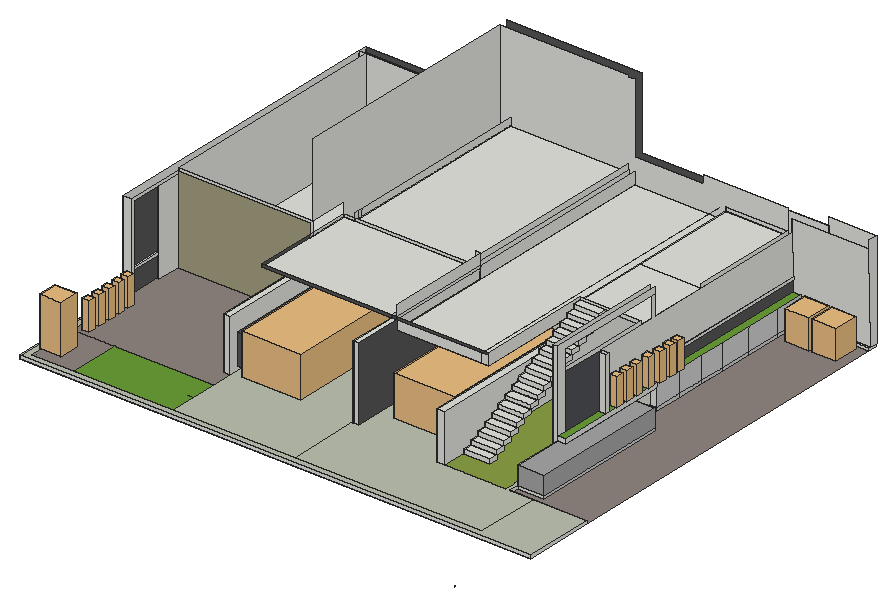
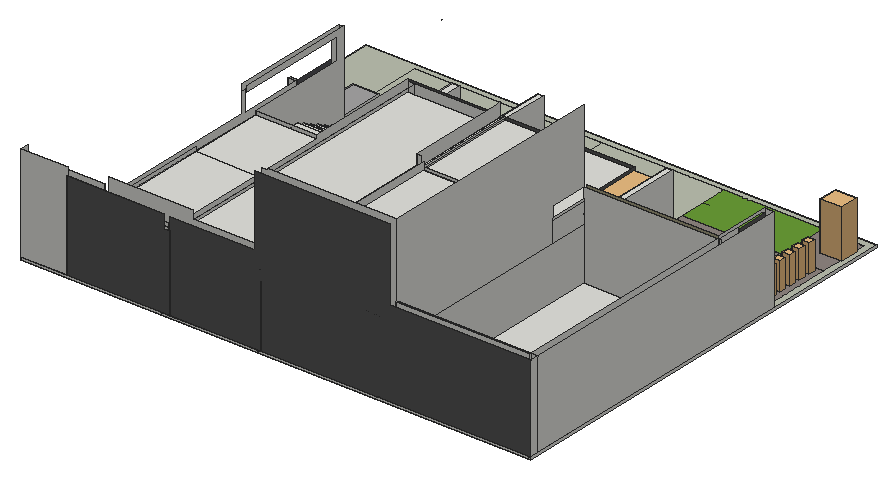
# SketchUp Ruby script. Lengths in inches.
U = 1.inch
M = Sketchup.active_model
def pt(a) = Geom::Point3d.new(a.map { |v| v * U })
def face(e, loops, mat)
  f = e.add_face(loops[0].map { |a| pt(a) })
  loops[1..].each { |l| e.add_face(l.map { |a| pt(a) }).erase! }
  f.material = f.back_material = mat if mat
  f
end
# faces: each face lists its corners as indices into pts; further lists are holes
def faces(e, pts, list, mat = nil) = list.each { |f| face(e, (f[0].is_a?(Array) ? f : [f]).map { |l| l.map { |i| pts[i] } }, mat) }
# xy, xz, yz: faces in a plane at the given z, y or x. An outline is a flat list of corners, or four numbers for a rectangle; further outlines are holes
def ring(l) = l.size == 4 ? [[l[0], l[1]], [l[2], l[1]], [l[2], l[3]], [l[0], l[3]]] : l.each_slice(2).to_a
def flat(e, list, mat, &to3) = list.each { |f| face(e, (f[0].is_a?(Array) ? f : [f]).map { |l| ring(l).map { |u, v| to3.(u, v) } }, mat) }
def xy(e, z, list, mat = nil) = flat(e, list, mat) { |x, y| [x, y, z] }
def xz(e, y, list, mat = nil) = flat(e, list, mat) { |x, z| [x, y, z] }
def yz(e, x, list, mat = nil) = flat(e, list, mat) { |y, z| [x, y, z] }
def lines(e, pts, list) = list.each { |a, b| e.add_line(pt(pts[a]), pt(pts[b])) }
# prism: a flat outline (further loops are holes) pulled along v
def prism(e, loops, v, mat = nil)
  f = face(e, loops, mat); d = Geom::Vector3d.new(v.map { |x| x * U })
  f.pushpull(f.normal.samedirection?(d) ? d.length : -d.length)
end
def box(e, o, s, mat = nil) = prism(e, [[o, [o[0] + s[0], o[1], o[2]], [o[0] + s[0], o[1] + s[1], o[2]], [o[0], o[1] + s[1], o[2]]]], [0, 0, s[2]], mat)
def at(x, y, z, deg = 0) = Geom::Transformation.translation(pt([x, y, z])) * Geom::Transformation.rotation(ORIGIN, Z_AXIS, deg.degrees)
def axes(o, x, y, z) = Geom::Transformation.new([*x, 0, *y, 0, *z, 0, *pt(o).to_a, 1])
def part(name) = M.definitions.add(name)
# library, detail: a bought-in or finely detailed component or shape, given as its bounding box
def library(name, o, s) = part(name).tap { |d| box(d.entities, o, s) }
def detail(e, o, s) = box(e.add_group.entities, o, s)
def put(e, d, t, mat = nil) = e.add_instance(d, t).tap { |i| i.material = mat if mat }
def group(e, t, mat = nil) = e.add_group.tap { |g| g.transformation = t; g.material = mat if mat }.entities
root = M.entities
M.materials.add("[Blinds Roman Hobbled Blue]").color = [81, 82, 87]
M.materials.add("[Carrera Marble]").color = [207, 207, 207]
M.materials.add("[Color M06]").color = [86, 86, 86]
M.materials.add("[Grass Dark Green]").color = [106, 157, 55]
M.materials.add("[Grass Light Green]").color = [138, 158, 69]
M.materials.add("[Groundcover Rock Crushed Multi]").color = [143, 133, 129]
M.materials.add("[Pavers with Grass Brick]").color = [187, 192, 176]
M.materials.add("[Stone Coursed Rough]").color = [165, 160, 130]
M.materials.add("[Stone Vein Gray]").color = [166, 165, 165]
c1 = library("PLANTS 75\#1",[-17.06,-18.11,0],[33.69,34.67,40.66])
c2 = library("bmw m6",[0,0,0],[74.56,175.18,49.66])
c3 = library("MERCEDES LIGHT",[-74.97,-97.73,0.18],[82.22,195.9,56.22])
c4 = library("araç",[-7.9,-14.14,0],[84.07,190.26,56.29])
c5 = part("Group\#4")
box(c5.entities,[0,0,0],[36,12,6])
c6 = library("PLANTS 75",[-17.8,-11.72,0],[29.52,26.34,67.21])
c7 = library("Plant Pot 02 - Garden Croton",[-1.84,-1.8,0],[9.84,9.84,38.82])
xy(root,0,[[710.71,0,710.77,0,710.83,0.04,710.85,0.0625,710.86,0.09,710.86,0.16,710.85,0.1875,710.83,0.21,710.77,0.25,710.71,0.25,710.65,0.21,710.63,0.1875,710.62,0.16,710.61,0.125,710.62,0.09,710.63,0.0625,710.65,0.04],[27.5625,99.87,27.5625,699.87,736.75,699.87,736.75,688.37,640,688.37,640,687.87,39.5625,687.87,39.5625,111.87,736.75,111.87,736.75,99.87],[39.5625,111.87,39.5625,687.87,640,687.87,640,440.86,629.0625,440.86,629.0625,403.96,665.5,403.96,665.5,211.52,629.0625,211.52,629.0625,198.37,736.75,198.37,736.75,111.87],[640,687.87,736.75,688.37]])
xy(root,0,[[629.0625,198.37,736.75,198.37,736.75,687.87,640,687.87,640,440.86,629.0625,440.86,629.0625,403.96,665.5,403.96,665.5,211.52,629.0625,211.52]],"[Groundcover Rock Crushed Multi]")
xy(root,3.4375,[[404.1875,699.87,415.125,700.56]])
xy(root,4,[[223,208.68,232,208.68,232,418.01,238,418.01,238,688.37,223,688.37],[403.0625,208.68,403.6875,688.37],[403.6875,208.68,410.3125,688.37],[629.0625,211.52,665.5,403.96],[27.5625,278.75,39.5625,278.75,39.5625,281.87,36.5625,281.87,36.5625,326.25,39.5625,326.25,39.5625,358.3125,36.5625,358.3125,36.5625,688.37,27.5625,688.37],
  [622.9375,281.31,629.0625,281.31,629.0625,440.86,640,440.86,640,688.37,622.9375,688.37],[36.5625,358.3125,223,364.3125],[36.5625,364.3125,223,688.37],[27.5625,688.37,27.5625,699.87,238,699.87,238,688.37,223,688.37,223,690.87,36.5625,690.87,36.5625,688.37],[36.5625,688.37,223,690.87],
  [238,688.37,401.5625,690.87],[401.5625,688.37,403.0625,690.87],[403.0625,688.37,403.6875,690.87],[403.0625,688.37,403.6875,699.87],[403.6875,688.37,404.1875,690.87],
  [404.1875,688.37,410.3125,699.87],[410.3125,688.37,415.125,699.87],[415.125,688.37,528.4375,699.87],[528.4375,688.37,537.4375,690.87],[537.4375,688.37,640,690.87],
  [640,688.37,662.375,690.87],[662.375,688.37,736.75,690.87],[238,690.87,401.5625,699.87],[401.5625,690.87,403.0625,699.87],[403.0625,690.87,403.6875,699.87],
  [403.6875,690.87,404.1875,699.87],[528.4375,690.87,537.4375,699.87],[537.4375,690.87,736.75,699.87],[27.5625,699.87,238,700.56],[238,699.87,238,700.43,351.24,700.43],
  [238,699.87,351.24,700.43,401.5625,700.43,401.5625,699.87],[401.5625,699.87,403.6875,700.43],[403.6875,699.87,404.1875,700.43],[404.1875,699.87,415.125,700.56],[415.125,699.87,528.4375,700.56],
  [528.4375,699.87,537.4375,700.56],[537.4375,699.87,736.75,700.56],[238,700.43,238,700.68,401.5625,700.68,351.24,700.43],[351.24,700.43,401.5625,700.68,401.5625,700.43],[401.5625,700.43,404.1875,700.68],
  [27.5625,700.56,238,700.68],[404.1875,700.56,415.125,700.68],[415.125,700.56,528.4375,700.68],[528.4375,700.56,537.4375,700.68],[537.4375,700.56,671.375,700.68]])
xy(root,4,[[95.3,108.87,232,180.0625]],"[Grass Dark Green]")
xy(root,4,[[538.22,198.37,622.9375,688.37]],"[Grass Light Green]")
xy(root,4,[[36.5625,108.87,95.3,180.0625],[36.5625,180.0625,232,180.0625,232,208.68,223,208.68,223,358.3125,39.5625,358.3125,39.5625,326.25,36.5625,326.25,36.5625,281.87,39.5625,281.87,39.5625,278.75,36.5625,278.75]],"[Groundcover Rock Crushed Multi]")
xy(root,4,[[27.5625,99.87,736.75,99.87,736.75,198.37,662.375,198.37,662.375,108.87,36.5625,108.87,36.5625,278.75,27.5625,278.75],[232,108.87,401.3125,108.87,401.3125,208.68,403.0625,208.68,403.0625,688.37,238,688.37,238,418.01,232,418.01],[401.3125,108.87,662.375,108.87,662.375,198.37,629.0625,198.37,629.0625,281.31,622.9375,281.31,622.9375,198.37,527.29,198.37,527.29,688.37,410.3125,688.37,410.3125,208.68,401.3125,208.68]],"[Pavers with Grass Brick]")
xy(root,4.1875,[[404.1875,699.87,528.4375,700.56]])
xy(root,10.27,[[232,219.93,239.75,400.37]])
xy(root,29.125,[[629.0625,281.31,640,325.03],[629.0625,325.03,640,403.96],[629.0625,403.96,640,440.86]])
xy(root,29.125,[[629.0625,211.52,665.5,211.52,665.5,403.96,640,403.96,640,281.31,629.0625,281.31]],"[Stone Vein Gray]")
xy(root,34.11,[[36.5625,281.87,39.5625,326.25]])
xy(root,34.7,[[629.0625,281.31,640,352.35],[629.0625,356.66,640,690.25]],"[Grass Dark Green]")
xy(root,37.14,[[36.5625,281.87,39.5625,326.25]])
xy(root,51.11,[[629.0625,356.66,631.0625,689.91]])
xy(root,52.52,[[232,219.93,239.75,400.37]],"[Color M06]")
xy(root,54.25,[[629.0625,356.66,631.0625,689.85]])
xy(root,69.25,[[527.29,198.37,538.22,688.37]])
xy(root,76,[[223,208.68,232,418.01]])
xy(root,92.625,[[403.0625,275.76,410.3125,420.51],[410.3125,275.76,537.4375,690.87],[403.0625,420.51,410.3125,421.2],[403.0625,421.2,410.3125,690.87],[403.0625,690.87,410.3125,699.87]])
xy(root,103.9375,[[537.4375,434.32,622.9375,538.51],[537.4375,538.51,622.9375,688.37]])
xy(root,105.3125,[[223,275.76,403.6875,418.01],[238,418.01,401.5625,690.87],[238,690.87,242.1875,690.87,242.1875,699.89,238,699.87],[242.1875,690.87,244.125,690.87,244.125,699.9,242.1875,699.89],[252.72,690.87,256.22,690.87,256.22,699.96,252.72,699.95]])
xy(root,105.6875,[[403.0625,208.68,403.6875,275.76],[403.6875,208.68,410.3125,275.76],[403.0625,275.76,403.6875,275.76,403.6875,275.77,403.27,418.01,403.26,420.51,403.0625,420.51],[403.9375,275.76,410.25,275.78,410.25,275.79,409.83,418.03,403.27,418.01,403.6875,275.77,403.9375,275.77],[403.6875,275.76,403.9375,275.77],
  [403.9375,275.76,410.25,275.78,410.25,275.79,403.9375,275.77],[403.9375,275.76,410.3125,275.76,410.3125,420.51,409.82,420.51,409.83,418.03,410.25,275.79,410.25,275.78],[403.6875,275.77,403.9375,275.77,410.25,275.79,409.83,418.03,403.27,418.01],[403.27,418.01,409.83,418.03,409.82,420.51,403.26,420.51],[403.26,420.51,409.82,421.2],
  [409.82,420.51,410.3125,421.2],[403.26,421.2,409.82,421.22,409.82,421.2]])
xz(root,99.87,[[27.5625,0,736.75,4]])
xz(root,198.37,[[629.0625,0,662.375,4],[662.375,0,736.75,4],[527.29,4,538.22,69.25]])
xz(root,208.68,[[223,4,232,76],[403.0625,4,403.6875,105.6875],[403.6875,4,410.3125,105.6875]])
xz(root,211.52,[[629.0625,0,665.5,4]])
xz(root,211.52,[[629.0625,4,665.5,29.125]],"[Stone Vein Gray]")
xz(root,219.93,[[232,10.27,239.75,52.52]],"[Color M06]")
xz(root,275.76,[[403.0625,92.625,410.3125,105.6875],[410.3125,92.625,528.4375,105.6875],[528.4375,92.625,537.4375,105.6875],[403.0625,105.3125,403.6875,105.6875]])
xz(root,275.76,[[223,105.3125,403.0625,105.3125,403.0625,105.6875,403.6875,105.6875,403.6875,109.0625,223,109.0625],[410.3125,105.6875,537.4375,109.0625]],"[Color M06]")
xz(root,278.75,[[27.5625,4,39.5625,124]])
xz(root,281.31,[[622.9375,4,629.0625,146.75],[629.0625,29.125,640,34.7]])
xz(root,281.87,[[36.5625,4,39.5625,34.11],[36.5625,37.14,39.5625,120.67]])
xz(root,326.25,[[36.5625,4,39.5625,34.11],[36.5625,37.14,39.5625,120.67]])
xz(root,352.35,[[629.0625,34.7,640,109.0625]])
xz(root,356.66,[[629.0625,34.7,629.0625,51.11,631.0625,51.11,631.0625,54.25,629.0625,54.25,629.0625,109.0625,640,109.0625,640,34.7]])
xz(root,358.3125,[[36.5625,4,39.5625,120.67]])
xz(root,358.3125,[[39.5625,4,223,124]],"[Stone Coursed Rough]")
xz(root,364.3125,[[36.5625,4,223,124]])
xz(root,400.37,[[232,10.27,239.75,52.52]])
xz(root,403.96,[[629.0625,0,665.5,4]])
xz(root,403.96,[[629.0625,4,665.5,29.125]],"[Stone Vein Gray]")
xz(root,418.01,[[232,4,238,4,238,105.3125,223,105.3125,223,76,232,76],[223,105.3125,238,109.0625],[238,105.3125,401.5625,109.0625],[401.5625,105.3125,403.6875,109.0625]])
xz(root,420.51,[[403.0625,92.625,410.3125,105.6875]])
xz(root,421.2,[[403.0625,92.625,410.3125,105.6875],[403.0625,105.6875,403.26,109.0625],[403.26,105.6875,410.3125,109.0625]])
xz(root,434.32,[[537.4375,103.9375,622.9375,109.0625]])
xz(root,440.86,[[629.0625,0,640,4],[629.0625,4,640,29.125]])
xz(root,688.37,[[640,0,662.375,4],[662.375,0,736.75,4],[27.5625,4,527.29,4,527.29,69.25,538.22,69.25,538.22,4,622.9375,4,622.9375,103.9375,537.4375,103.9375,537.4375,109.0625,622.9375,109.0625,622.9375,138.0625,506.53,138.0625,506.53,127,410.3125,127,410.3125,224.0625,401.5625,224.0625,401.5625,225.8125,223,225.8125,223,124,27.5625,124],[537.4375,103.9375,622.9375,109.0625]])
xz(root,690.87,[[36.5625,4,223,124],[238,4,403.6875,4,403.6875,92.625,403.0625,92.625,403.0625,105.3125,238,105.3125],[403.6875,4,404.1875,92.625],[528.4375,4,537.4375,92.625],[403.0625,92.625,403.6875,105.3125],
  [404.1875,92.625,404.1875,105.3125,403.0625,105.3125,403.0625,105.6875,410.3125,105.6875,410.3125,92.625],[403.6875,92.625,404.1875,105.3125],[410.3125,92.625,426.77,105.6875],[426.77,92.625,437.7,105.6875],[437.7,92.625,528.4375,105.6875],
  [528.4375,92.625,537.4375,109.0625],[238,105.3125,242.1875,115.375],[242.1875,105.3125,244.125,115.375],[244.125,105.3125,252.72,115.375],[252.72,105.3125,256.22,115.375],
  [256.22,105.3125,401.5625,115.375],[403.0625,105.6875,410.3125,109.0625],[410.3125,105.6875,426.77,109.0625],[426.77,105.6875,437.7,109.0625],[437.7,105.6875,528.4375,109.0625]])
xz(root,699.87,[[27.5625,0,27.5625,4,404.1875,4,404.1875,3.4375,415.125,3.4375,415.125,4,736.75,4,736.75,0],[404.1875,3.4375,404.78,4],[404.78,3.4375,405.72,4],[405.72,3.4375,410.3125,4],[410.3125,3.4375,415.125,4],
  [403.0625,4,404.1875,4.1875],[404.1875,4,404.78,4.1875],[404.78,4,405.72,4.1875],[405.72,4,410.3125,4.1875],[410.3125,4,528.4375,4.1875],
  [403.0625,4.1875,404.1875,92.625],[404.1875,4.1875,410.3125,92.625],[404.1875,92.625,410.3125,92.625,410.3125,115.375,401.5625,115.375,401.5625,105.3125,404.1875,105.3125]])
xz(root,700.56,[[404.1875,3.4375,415.125,4],[404.1875,4,415.125,4.1875],[415.125,4,528.4375,4.1875],[528.4375,4,537.4375,109.0625],[537.4375,4,671.375,127],
  [671.375,4,736.75,138.0625]])
xz(root,700.68,[[27.5625,4,27.5625,124,223,124,223,225.8125,410.3125,225.8125,410.3125,127,528.4375,127,528.4375,109.0625,537.4375,109.0625,537.4375,127,671.375,127,671.375,4]],"[Color M06]")
yz(root,27.5625,[[99.87,0,699.87,4],[278.75,4,688.37,124],[688.37,4,700.56,124],[700.56,4,700.68,124]])
yz(root,36.5625,[[364.3125,4,690.87,124]])
yz(root,36.5625,[[281.87,4,326.25,34.11],[281.87,37.14,326.25,120.67]],"[Color M06]")
yz(root,39.5625,[[278.75,4,281.87,4,281.87,120.67,358.3125,120.67,358.3125,124,278.75,124],[326.25,4,358.3125,120.67],[281.87,34.11,326.25,37.14]])
yz(root,223,[[208.68,4,358.3125,76],[358.3125,4,364.3125,76],[364.3125,4,690.87,76],[358.3125,76,364.3125,105.3125],[364.3125,76,418.01,105.3125],
  [418.01,76,418.01,123.8125,364.3125,123.8125,364.3125,225.8125,688.37,225.8125,688.37,124,690.87,124,690.87,76],[358.3125,105.3125,364.3125,109.0625],[364.3125,105.3125,418.01,109.0625]])
yz(root,223,[[275.76,105.3125,358.3125,109.0625]],"[Color M06]")
yz(root,232,[[[208.68,4,418.01,76],[219.93,10.27,400.37,52.52]]])
yz(root,238,[[418.01,4,690.87,105.3125],[690.87,4,699.87,105.3125],[418.01,105.3125,424.01,115.375],[424.01,105.3125,430.01,115.375],[430.01,105.3125,690.87,115.375]])
yz(root,239.75,[[219.93,10.27,400.37,52.52]],"[Color M06]")
yz(root,401.5625,[[418.01,105.3125,690.87,115.375]])
yz(root,403.0625,[[208.68,4,208.68,105.6875,275.76,105.6875,275.76,92.625,699.87,92.625,699.87,4],[275.76,92.625,420.51,105.6875],[421.2,92.625,690.87,109.0625]])
yz(root,403.6875,[[275.76,105.3125,275.76,105.6875,275.77,105.6875,275.77,109.0625,418.01,109.0625,418.01,105.3125]])
yz(root,404.1875,[[699.87,3.4375,700.43,4],[700.43,3.4375,700.56,4],[699.87,4,700.43,4.1875],[700.43,4,700.56,4.1875]])
yz(root,410.25,[[275.78,105.6875,275.79,109.0625]])
yz(root,410.3125,[[275.76,92.625,420.51,105.6875],[420.51,92.625,421.2,105.6875],[421.2,92.625,690.87,109.0625],[690.87,92.625,699.87,109.0625],[275.76,105.6875,420.51,109.0625],
  [420.51,105.6875,421.2,109.0625]])
yz(root,410.3125,[[208.68,4,699.87,4,699.87,92.625,275.76,92.625,275.76,105.6875,208.68,105.6875]],"[Color M06]")
yz(root,415.125,[[699.87,3.4375,700.56,4]])
yz(root,527.29,[[198.37,4,688.37,69.25]])
yz(root,528.4375,[[690.87,4,699.87,4,690.87,92.625],[699.87,4,699.87,4.1875,700.56,4.1875,700.56,109.0625,690.87,109.0625,690.87,92.625],[699.87,4,700.56,4.1875]])
yz(root,537.4375,[[275.76,92.625,688.37,92.625,688.37,103.9375,434.32,103.9375,434.32,109.0625,275.76,109.0625],[688.37,92.625,690.87,109.0625]])
yz(root,538.22,[[198.37,4,688.37,69.25]])
yz(root,622.9375,[[281.31,4,281.31,146.75,449.72,146.75,449.72,138.66,293.21,138.66,293.21,109.0625,434.32,109.0625,434.32,103.9375,688.37,103.9375,688.37,4],[538.51,103.9375,688.37,109.0625]])
yz(root,629.0625,[[198.37,0,211.52,4],[403.96,0,440.86,4],[211.52,4,281.31,29.125],[281.31,4,403.96,29.125],[403.96,4,440.86,29.125],
  [281.31,34.7,293.21,34.7,293.21,138.66,449.72,138.66,449.72,146.75,281.31,146.75],[356.66,54.25,689.85,54.25,688.37,127,688.37,109.0625,449.72,109.0625,449.72,138.66,445.9375,138.66,445.9375,109.0625,356.66,109.0625]])
yz(root,629.0625,[[293.21,34.7,352.35,109.0625]],"[Blinds Roman Hobbled Blue]")
yz(root,629.0625,[[356.66,34.7,690.25,34.7,689.91,51.11,356.66,51.11]],"[Color M06]")
yz(root,631.0625,[[356.66,51.11,689.91,51.11,689.85,54.25,356.66,54.25]])
yz(root,640,[[281.31,29.125,440.86,34.7],[352.35,34.7,356.66,109.0625]])
yz(root,640,[[440.86,0,479.17,4],[479.17,0,517.36,4],[517.36,0,554.04,4],[554.04,0,599.36,4],[599.36,0,647.79,4],
  [647.79,0,688.37,4],[440.86,4,479.17,34.7],[479.17,4,517.36,34.7],[517.36,4,554.04,34.7],[554.04,4,599.36,34.7],
  [599.36,4,647.79,34.7],[647.79,4,690.87,4,690.25,34.7,647.79,34.7]],"[Carrera Marble]")
yz(root,665.5,[[211.52,0,403.96,4]],"[Carrera Marble]")
yz(root,665.5,[[211.52,4,403.96,29.125]],"[Stone Vein Gray]")
yz(root,671.375,[[700.56,4,700.68,127]])
yz(root,736.75,[[99.87,0,198.37,4],[688.37,0,699.87,4],[690.87,4,700.56,4,700.56,138.0625,688.37,138.0625,688.37,127]])
p = [[629.0625,688.37,127],[629.0625,689.85,54.25],[631.0625,689.85,54.25],[631.0625,689.91,51.11],[629.0625,689.91,51.11],[629.0625,690.25,34.7],
  [640,690.25,34.7],[640,690.87,4],[662.375,690.87,4],[736.75,690.87,4],[736.75,688.37,127],[537.4375,690.87,92.625],
  [528.4375,690.87,92.625],[528.4375,699.87,4],[537.4375,699.87,4],[403.6875,275.76,109.0625],[403.6875,275.76,105.6875],[403.9375,275.76,105.6875],
  [410.25,275.78,105.6875],[410.25,275.78,109.0625],[403.6875,275.77,105.6875],[403.6875,275.77,109.0625],[410.25,275.79,109.0625],[410.25,275.79,105.6875],
  [403.9375,275.77,105.6875],[410.25,275.78,124.25],[409.83,418.03,105.6875],[409.82,420.51,105.6875],[409.82,421.2,105.6875],[409.82,421.22,105.6875],
  [409.82,421.22,124.25],[409.82,421.2,124.25],[409.82,420.51,124.25],[410.23,281.71,124.25],[403.26,421.2,109.0625],[403.26,421.2,124.25],
  [403.26,421.2,105.6875],[39.5625,687.87,0],[39.5625,687.87,4],[39.5625,111.87,0],[39.5625,111.87,4],[223,699.87,76],
  [223,690.87,76],[403.27,418.01,109.0625],[403.27,418.01,105.6875],[528.4375,275.76,105.6875],[528.4375,690.87,105.6875],[403.6875,700.43,105.3125],
  [404.1875,700.43,105.3125],[403.6875,700.56,105.3125],[404.1875,700.56,105.3125],[256.22,699.96,105.3125],[256.22,700.68,105.3125],[244.125,699.9,105.3125],
  [244.125,700.68,105.3125],[242.1875,699.89,105.3125],[242.1875,700.68,105.3125],[238,699.87,105.3125],[238,700.68,105.3125],[404.1875,700.43,4.1875],
  [252.72,699.95,105.3125],[252.72,700.56,105.3125],[39.5625,144.47,0],[232,144.47,4]]
faces(root,p,[[0,1,2,3,4,5,6,7,8,9,10],[11,12,13,14],[20,21,22,23,24],[25,19,22,23,26,27,28,29,30,31,32,33],[34,35,30,29,36]])
faces(root,p,[[15,16,17,18,19]],"[Color M06]")
lines(root,p,[[37,38],[39,40],[41,42],[43,44],[45,46],[47,48],[49,50],[51,52],[53,54],[55,56],[57,58],[59,48],
  [60,61],[62,63]])
put(root,c1,at(706.32,666.02,0))
put(root,c1,at(668.26,666.02,0))
put(root,c2,axes([431.36,244.79,4],[1.12,0,0],[0,1.05539,0],[0,0,1.12246]))
put(root,c3,at(251.49,311.16,3.82,180))
put(root,c4,at(324.65,393.5625,4))
g1 = group(root,at(538.29,230.32,4))
put(g1,c5,at(1.75,24,12))
g2 = group(g1,at(1.25,48,24))
box(g2,[0,0,0],[36,12,6])
g3 = group(g1,at(0.75,72,36))
box(g3,[0,0,0],[36,12,6])
put(g1,c5,at(0.25,96,48))
put(g1,c5,at(2,0,0))
put(g1,c5,at(0,108,54))
g4 = group(g1,at(2,12,6))
box(g4,[0,0,0],[36,12,6])
put(g1,c5,at(1.5,36,18))
put(g1,c5,at(1,60,30))
put(g1,c5,at(0.5,84,42))
put(root,c6,at(52.1875,137.32,4))
put(root,c7,at(45.96,188.19,4))
put(root,c7,at(45.96,205.19,4))
put(root,c7,at(45.96,222.19,4))
put(root,c7,at(45.96,239.19,4))
put(root,c7,at(45.96,256.19,4))
put(root,c7,at(632.92,371.65,35.4))
put(root,c7,at(632.92,388.65,35.4))
put(root,c7,at(632.92,405.65,35.4))
put(root,c7,at(632.92,426.33,35.4))
put(root,c7,at(635.17,443.33,35.4))
put(root,c7,at(635.17,460.33,35.4))
put(root,c7,at(635.17,474.65,35.4))
put(root,c5,at(538.29,350.32,64))
put(root,c5,at(538.29,362.32,70))
put(root,c5,at(538.29,374.32,76))
put(root,c5,at(538.29,386.32,82))
put(root,c5,at(538.29,398.32,88))
put(root,c5,at(538.29,410.32,94))
put(root,c5,at(538.29,422.32,100))
